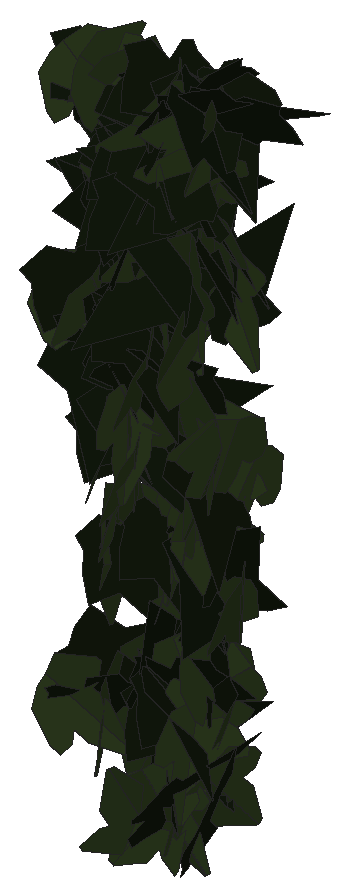
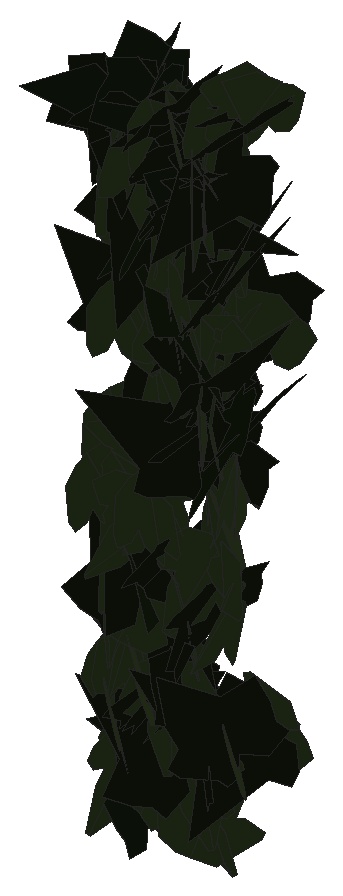
# SketchUp Ruby script. Lengths in inches.
U = 1.inch
M = Sketchup.active_model
def pt(a) = Geom::Point3d.new(a.map { |v| v * U })
def face(e, loops, mat)
  f = e.add_face(loops[0].map { |a| pt(a) })
  loops[1..].each { |l| e.add_face(l.map { |a| pt(a) }).erase! }
  f.material = f.back_material = mat if mat
  f
end
# faces: each face lists its corners as indices into pts; further lists are holes
def faces(e, pts, list, mat = nil) = list.each { |f| face(e, (f[0].is_a?(Array) ? f : [f]).map { |l| l.map { |i| pts[i] } }, mat) }
# xy, xz, yz: faces in a plane at the given z, y or x. An outline is a flat list of corners, or four numbers for a rectangle; further outlines are holes
def ring(l) = l.size == 4 ? [[l[0], l[1]], [l[2], l[1]], [l[2], l[3]], [l[0], l[3]]] : l.each_slice(2).to_a
def flat(e, list, mat, &to3) = list.each { |f| face(e, (f[0].is_a?(Array) ? f : [f]).map { |l| ring(l).map { |u, v| to3.(u, v) } }, mat) }
def xy(e, z, list, mat = nil) = flat(e, list, mat) { |x, y| [x, y, z] }
def xz(e, y, list, mat = nil) = flat(e, list, mat) { |x, z| [x, y, z] }
def yz(e, x, list, mat = nil) = flat(e, list, mat) { |y, z| [x, y, z] }
def lines(e, pts, list) = list.each { |a, b| e.add_line(pt(pts[a]), pt(pts[b])) }
# prism: a flat outline (further loops are holes) pulled along v
def prism(e, loops, v, mat = nil)
  f = face(e, loops, mat); d = Geom::Vector3d.new(v.map { |x| x * U })
  f.pushpull(f.normal.samedirection?(d) ? d.length : -d.length)
end
def box(e, o, s, mat = nil) = prism(e, [[o, [o[0] + s[0], o[1], o[2]], [o[0] + s[0], o[1] + s[1], o[2]], [o[0], o[1] + s[1], o[2]]]], [0, 0, s[2]], mat)
def at(x, y, z, deg = 0) = Geom::Transformation.translation(pt([x, y, z])) * Geom::Transformation.rotation(ORIGIN, Z_AXIS, deg.degrees)
def axes(o, x, y, z) = Geom::Transformation.new([*x, 0, *y, 0, *z, 0, *pt(o).to_a, 1])
def part(name) = M.definitions.add(name)
# library, detail: a bought-in or finely detailed component or shape, given as its bounding box
def library(name, o, s) = part(name).tap { |d| box(d.entities, o, s) }
def detail(e, o, s) = box(e.add_group.entities, o, s)
def put(e, d, t, mat = nil) = e.add_instance(d, t).tap { |i| i.material = mat if mat }
def group(e, t, mat = nil) = e.add_group.tap { |g| g.transformation = t; g.material = mat if mat }.entities
root = M.entities
M.materials.add("efeu1").color = [18, 25, 13]
M.materials.add("efeu2").color = [43, 57, 29]
c1 = part("ivyleaf_9")
p = [[1.54,2.16,1.25],[1.36,2.04,1.19],[-0.21,0.99,0.68],[-0.71,1.11,0.82],[-0.85,0.86,0.67],[-0.8,0.17,0.21],
  [-0.9,-0.01,0.1],[-0.67,-0.16,-0.02],[-0.08,-0.08,-0.05],[-0.03,-0.6,-0.4],[0.65,-0.88,-0.66],[0.83,-0.6,-0.49],
  [1.29,-0.42,-0.43],[1.8125,-0.07,-0.26],[1.21,0.44,0.15]]
faces(c1.entities,p,[[0,1,2,3,4,5,6,7,8,9,10,11,12,13,14]],"efeu1")
c2 = part("ivyleaf_10")
p = [[0,0.5,-0.03],[-0.0625,2.02,-0.43],[-0.19,2.01,-0.46],[-0.54,1.05,-0.29],[-0.52,0.625,-0.18],[-0.83,0.76,-0.28],
  [-1.16,0.64,-0.33],[-1.15,0.33,-0.24],[-0.77,-0.39,0.02],[-0.3,-0.51,0.16],[0.04,-0.48,0.23],[-0.02,2.01,-0.4375],
  [-0.06,2.01,-0.43],[0.04,-0.49,0.23],[0.67,-0.49,0.14],[1.38,0.36,-0.2],[1.375,0.51,-0.24],[0.81,0.65,-0.19],
  [0.62,0.59,-0.15],[0.6,1.09,-0.28],[0.5,1.23,-0.31]]
faces(c2.entities,p,[[0,1,2,3,4,5,6,7,8,9,10],[11,12,0,13,14,15,16,17,18,19,20]],"efeu2")
put(root,c1,axes([26.85,224.39,219.23],[0.01117,-0.47465,0.1568],[0.04061,-0.15546,-0.47348],[0.49822,0.02332,0.03508]))
put(root,c1,axes([27.04,224.61,221.03],[-0.15188,-0.0856,0.46862],[-0.11517,-0.47067,-0.1233],[0.46224,-0.14539,0.12325]))
put(root,c1,axes([26.95,224.09,215.43],[0.39928,0.30016,-0.02189],[-0.01757,-0.01306,-0.49952],[-0.30044,0.39967,0.00012]))
put(root,c1,axes([27.18,224.76,220.63],[-0.0054,-0.49964,0.01817],[0.00355,0.01813,0.49966],[-0.49996,0.00553,0.00335]))
put(root,c2,axes([27.07,224.33,216.95],[0.09969,-0.16852,-0.46007],[0.02423,0.47062,-0.16713],[0.48936,0.01103,0.102]))
put(root,c2,axes([26.68,223.98,215.4],[0.18664,0.05922,0.46006],[0.44103,0.13102,-0.19578],[-0.14374,0.47888,-0.00333]))
put(root,c2,axes([27.21,224.04,218.6],[0.07906,-0.26335,-0.41761],[-0.14047,0.39345,-0.27471],[0.47331,0.16076,-0.01177]))
put(root,c2,axes([26.77,223.9375,220.31],[0.2244,0.20804,0.39543],[0.29999,0.25778,-0.30587],[-0.33113,0.37452,-0.00912]))
put(root,c1,axes([27.27,224.71,219.45],[-0.16065,-0.47331,-0.01309],[0.01351,-0.0184,0.49948],[-0.47329,0.16013,0.0187]))
put(root,c1,axes([27.02,224.31,219.47],[0.40451,-0.11818,-0.26909],[-0.25817,0.07588,-0.42142],[0.14044,0.47987,0.00036]))
put(root,c1,axes([26.85,224.47,222.93],[0.08992,-0.48476,-0.0832],[0.07638,0.09732,-0.48445],[0.48588,0.07441,0.09155]))
put(root,c2,axes([26.92,223.96,223.06],[0.20217,0.37365,0.26366],[0.13517,0.22656,-0.42473],[-0.43687,0.24302,-0.0094]))
put(root,c2,axes([26.97,224.49,215.43],[0.2392,-0.318,0.30276],[0.20685,-0.22249,-0.39713],[0.38729,0.31524,0.02511]))
put(root,c1,axes([26.97,224.41,222.48],[0.41401,0.27531,0.05291],[0.05261,0.0164,-0.49695],[-0.27537,0.41705,-0.01538]))
put(root,c1,axes([27.01,224.29,221.35],[0.32908,-0.29569,-0.23296],[-0.17513,0.15365,-0.44241],[0.33322,0.37277,-0.00245]))
put(root,c2,axes([27.14,224,223.04],[0.03905,0.34792,0.35697],[-0.06235,0.35866,-0.34275],[-0.49456,-0.01775,0.0714]))
put(root,c1,axes([26.86,224.59,215.36],[-0.06324,-0.0071,0.49593],[0.49593,-0.00852,0.06312],[0.00755,0.49988,0.00812]))
put(root,c2,axes([27.15,223.96,220.41],[-0.05576,-0.45222,-0.20587],[0.08827,0.19486,-0.45193],[0.48898,-0.08675,0.0581]))
put(root,c2,axes([27.23,224.39,222.96],[-0.12269,-0.48418,-0.02274],[0.01304,0.02015,-0.49942],[0.48454,-0.12314,0.00768]))
put(root,c2,axes([27.11,224.31,217.375],[0.24025,-0.43764,0.02742],[-0.00015,0.03118,0.49903],[-0.4385,-0.23979,0.01485]))
put(root,c2,axes([27.18,224.18,219.97],[0.12548,0.34493,-0.33952],[0.05452,0.33844,0.36399],[0.48092,-0.12837,0.04733]))
put(root,c2,axes([27.1875,224.36,218.49],[-0.40365,0.29443,-0.01956],[0.01995,-0.00583,-0.49957],[-0.2944,-0.40408,-0.00704]))
put(root,c1,axes([26.99,223.91,220.76],[-0.03728,-0.1951,-0.45885],[0.14823,0.43499,-0.197],[0.47607,-0.15072,0.0254]))
put(root,c2,axes([27.37,224.56,219.68],[0.14882,-0.29129,-0.37816],[-0.15788,0.34378,-0.32694],[0.45048,0.21671,0.01034]))
put(root,c1,axes([27.07,224.55,217.21],[0.14098,-0.38613,-0.28466],[-0.06576,0.27834,-0.41013],[0.47519,0.15308,0.02769]))
put(root,c2,axes([27.2,224.64,217.57],[-0.47066,0.02713,-0.16655],[0.16675,-0.00077,-0.47137],[-0.02584,-0.49926,-0.00832]))
put(root,c1,axes([27.69,224.57,221.62],[-0.31695,0.07509,0.37935],[-0.3678,0.09296,-0.3257],[-0.11944,-0.48551,-0.00369]))
put(root,c2,axes([27.46,224.375,222.32],[0.10723,-0.23008,-0.43077],[-0.18386,0.38957,-0.25384],[0.45244,0.21284,-0.00106]))
put(root,c2,axes([27.34,224.65,222.26],[0.18297,-0.41234,-0.21564],[-0.02654,0.22209,-0.44718],[0.46456,0.17509,0.05938]))
put(root,c2,axes([27.53,224.14,221.58],[-0.43573,-0.03493,0.24274],[-0.23476,-0.08372,-0.43345],[0.07092,-0.4917,0.05656]))
put(root,c2,axes([27.43,224.72,220.42],[-0.37069,-0.33552,-0.00391],[0.00268,0.00286,-0.49998],[0.33553,-0.3707,-0.00032]))
put(root,c2,axes([27.13,224.6,219.23],[0.12946,-0.18409,0.44649],[0.35029,-0.28243,-0.21802],[0.33247,0.36925,0.05584]))
put(root,c2,axes([27.6,224.45,214.96],[-0.43721,-0.08452,0.22738],[-0.22603,-0.0282,-0.4451],[0.08806,-0.492,-0.01354]))
put(root,c1,axes([27.47,224.68,221.95],[-0.30706,-0.36456,0.15104],[-0.06968,-0.13828,-0.47542],[0.38841,-0.31301,0.03411]))
put(root,c1,axes([27.24,224.49,220.04],[0.24011,0.38946,0.20166],[-0.09867,-0.17604,0.45746],[0.42733,-0.25948,-0.00768]))
put(root,c1,axes([27.38,224.7,221.93],[-0.1233,-0.48443,-0.01097],[0.00351,0.01043,-0.49988],[0.48455,-0.12335,0.00083]))
put(root,c1,axes([27.14,224.02,219.74],[0.14993,-0.00016,0.47699],[0.46626,0.10549,-0.14652],[-0.10059,0.48874,0.03178]))
put(root,c2,axes([27.6,224.29,213.94],[-0.31895,-0.30639,-0.23322],[-0.14845,-0.18158,0.44158],[-0.35529,0.35093,0.02487]))
put(root,c1,axes([27.26,224.33,218.83],[-0.07244,-0.21034,-0.44778],[0.24746,0.37647,-0.21687],[0.42839,-0.25304,0.04955]))
put(root,c1,axes([27.74,224.66,220.78],[-0.30694,0.38374,-0.09236],[0.0627,-0.06812,-0.49135],[-0.38969,-0.31322,-0.0063]))
put(root,c2,axes([27.57,224.55,222.18],[0.43746,-0.22631,-0.08611],[-0.07205,0.04811,-0.49244],[0.23117,0.44325,0.00948]))
put(root,c1,axes([27.34,224.35,218.97],[0.08608,-0.41446,-0.2661],[0.03378,0.27447,-0.41656],[0.49137,0.05374,0.07525]))
put(root,c1,axes([27.76,223.86,221.32],[-0.16232,0.11742,-0.45811],[-0.3551,0.28962,0.20006],[0.31234,0.3903,-0.01063]))
put(root,c1,axes([27.47,224.74,222.625],[-0.1058,-0.48794,-0.02681],[0.00877,0.02553,-0.49927],[0.4886,-0.10612,0.00316]))
put(root,c2,axes([27.61,224,218.45],[0.11883,-0.46018,-0.15528],[0.00502,0.16101,-0.47334],[0.48565,0.11093,0.04288]))
put(root,c1,axes([27.75,224.34,222.58],[-0.42684,0.21247,-0.15055],[0.13313,-0.07039,-0.47678],[-0.2238,-0.4471,0.00352]))
put(root,c2,axes([27.73,224.61,215.88],[-0.48549,-0.0978,0.06878],[-0.06745,-0.01346,-0.49525],[0.09872,-0.49016,-0.00012]))
put(root,c2,axes([27.58,224.05,219.09],[0.07016,0.47942,-0.12341],[-0.03957,-0.11881,-0.48406],[-0.49347,0.07769,0.02127]))
put(root,c2,axes([27.68,224.54,217.03],[0.28528,-0.39847,-0.09918],[-0.05978,0.07917,-0.49006],[0.40625,0.29147,-0.00247]))
put(root,c2,axes([27.68,224.68,220.875],[0.36148,-0.31601,-0.13952],[-0.05411,0.14766,-0.47463],[0.34118,0.35823,0.07255]))
put(root,c2,axes([27.61,224.89,220.81],[0.0394,-0.16562,0.47013],[0.10887,-0.45735,-0.17024],[0.48641,0.11578,0.00002]))
put(root,c2,axes([27.73,224.05,219.65],[0.09976,-0.42101,-0.2506],[-0.04747,0.24623,-0.43257],[0.48764,0.11009,0.00916]))
put(root,c1,axes([27.36,224.56,215.13],[-0.03342,-0.01638,-0.49861],[0.49822,-0.02689,-0.03251],[-0.02575,-0.49901,0.01812]))
put(root,c1,axes([27.59,224.55,215.7],[0.08273,0.26611,0.41514],[-0.16662,-0.38109,0.27749],[0.4641,-0.18426,0.02563]))
put(root,c2,axes([27.41,224.6875,220.49],[0.24588,-0.20678,0.38313],[0.34647,-0.1735,-0.316],[0.26363,0.42088,0.05797]))
put(root,c2,axes([27.84,224.19,214.32],[0.41234,-0.12911,-0.25162],[-0.24284,0.06635,-0.432],[0.14494,0.47847,-0.00799]))
put(root,c1,axes([27.51,224.27,220.16],[0.10713,-0.4709,-0.12954],[-0.00593,0.13136,-0.4824],[0.48835,0.10489,0.02256]))
put(root,c2,axes([27.73,224.51,222.79],[0.23082,-0.44348,-0.00653],[-0.00185,0.0064,-0.49996],[0.44353,0.23083,0.00132]))
put(root,c2,axes([27.86,224.24,222.31],[-0.37407,-0.3261,0.06105],[-0.04322,-0.04332,-0.49624],[0.32894,-0.37654,0.00423]))
put(root,c1,axes([27.89,224.13,219.61],[0.2048,0.31369,-0.33114],[-0.18044,-0.27767,-0.37462],[-0.41893,0.27295,-0.00053]))
put(root,c1,axes([27.375,224.67,218.78],[0.10284,-0.03814,0.48782],[0.47965,-0.09071,-0.10821],[0.09676,0.49022,0.01793]))
put(root,c1,axes([27.64,224.33,222.17],[-0.08263,-0.42112,-0.25658],[0.03457,0.25457,-0.42895],[0.49191,-0.08863,-0.01295]))
put(root,c2,axes([27.84,224.83,218.28],[-0.17138,-0.4468,0.14489],[0.00794,-0.15697,-0.47466],[0.46964,-0.16039,0.0609]))
put(root,c2,axes([28.03,224.4,220.84],[0.16934,-0.18519,-0.43247],[-0.22363,0.3727,-0.24716],[0.4139,0.27713,0.0434]))
put(root,c1,axes([27.67,224.53,217.57],[0.09946,-0.44972,-0.19458],[-0.03311,0.19193,-0.46051],[0.48889,0.10449,0.00839]))
put(root,c1,axes([27.65,224.61,222.99],[0.10473,-0.47967,-0.0946],[-0.00259,0.0962,-0.49065],[0.4889,0.10326,0.01767]))
put(root,c1,axes([27.72,224.68,222.73],[-0.14991,-0.47105,-0.07511],[0.10029,0.04585,-0.48769],[0.46634,-0.16128,0.08074]))
put(root,c1,axes([28.09,224.23,220.9],[-0.47101,-0.13344,0.10171],[-0.09635,-0.03302,-0.48952],[0.13736,-0.48073,0.00539]))
put(root,c2,axes([27.84,224.53,218.5],[-0.36173,-0.34361,0.03299],[0.02646,0.02004,0.4989],[-0.34417,0.36267,0.00369]))
put(root,c2,axes([27.92,224.1875,221.05],[-0.24814,-0.43206,-0.04187],[0.01715,0.03843,-0.49823],[0.43374,-0.2487,-0.00425]))
put(root,c2,axes([27.93,224.59,222.71],[-0.06891,-0.48036,0.12045],[0.01082,-0.12304,-0.4845],[0.49511,-0.06417,0.02735]))
put(root,c2,axes([27.96,224.29,219.4375],[-0.47465,0.15718,-0.00058],[0.0002,-0.00122,-0.5],[-0.15718,-0.47465,0.0011]))
put(root,c1,axes([27.5625,224.68,215.02],[0.38011,0.24524,-0.213],[0.17405,0.12305,0.45229],[0.27426,-0.41799,0.00818]))
put(root,c1,axes([27.95,224.52,221.69],[0.27643,0.41421,-0.04487],[-0.02059,-0.0402,-0.49796],[-0.41613,0.27715,-0.00517]))
put(root,c2,axes([28.01,224.68,222.3],[-0.28969,-0.40566,0.03897],[0.02606,-0.06615,-0.49492],[0.4067,-0.28471,0.05947]))
put(root,c1,axes([27.82,224.08,221.75],[-0.10442,-0.39438,-0.28907],[0.06537,0.28168,-0.4079],[0.48459,-0.12298,-0.00727]))
put(root,c1,axes([28.15,224.36,222.94],[0.02001,0.4946,-0.07051],[-0.02127,-0.06966,-0.49467],[-0.49915,0.0228,0.01825]))
put(root,c1,axes([27.85,224.4,215.75],[0.18587,-0.4069,-0.22336],[-0.0869,0.20584,-0.4473],[0.45596,0.2051,0.0058]))
put(root,c2,axes([28.17,224.77,216.59],[-0.44103,-0.14302,-0.18718],[-0.17109,-0.07861,0.46319],[-0.16192,0.47262,0.0204]))
put(root,c2,axes([27.96,224.42,217.8],[0.41058,-0.27437,0.07839],[0.06825,-0.03894,-0.49379],[0.27707,0.41618,0.00547]))
put(root,c1,axes([28.125,224.63,221.86],[-0.31371,-0.30816,0.23797],[-0.1029,-0.22911,-0.43234],[0.3755,-0.32023,0.08033]))
put(root,c1,axes([27.89,224.42,215.64],[0.01016,-0.36796,-0.33838],[-0.00999,0.33823,-0.3681],[0.4998,0.01424,-0.00048]))
put(root,c1,axes([28.33,224.41,215.74],[0.01955,-0.04863,0.49725],[-0.29553,0.40011,0.05075],[-0.40284,-0.29589,-0.0131]))
put(root,c1,axes([28.45,224.16,222.09],[-0.29052,0.1168,0.38982],[-0.39346,0.04161,-0.30571],[-0.10386,-0.48438,0.06773]))
put(root,c2,axes([28.13,224.93,220.57],[-0.20779,-0.40735,0.20221],[-0.02015,-0.21385,-0.45151],[0.45433,-0.19579,0.07246]))
put(root,c2,axes([27.79,224.61,220.47],[0.38144,-0.07993,0.31323],[0.30755,-0.05952,-0.38971],[0.09959,0.48997,0.00376]))
put(root,c2,axes([28.22,224.55,216.13],[-0.35907,-0.31419,0.14951],[-0.10017,-0.1124,-0.47679],[0.33322,-0.37236,0.01777]))
put(root,c2,axes([27.88,224.12,214.59],[-0.39389,0.05915,-0.30224],[0.286,-0.11177,-0.3946],[-0.11425,-0.48374,0.05422]))
put(root,c1,axes([28.03,224.2,216.02],[0.41721,0.24579,-0.1246],[-0.10665,-0.06443,-0.48422],[-0.25409,0.43062,-0.00133]))
put(root,c1,axes([28.35,224.27,216.91],[-0.06569,0.27643,0.41142],[-0.10781,0.39712,-0.28403],[-0.4838,-0.12602,0.00743]))
put(root,c1,axes([27.8125,224.45,215.61],[0.20332,-0.40448,0.21226],[0.11442,-0.17983,-0.45229],[0.44223,0.23249,0.01944]))
put(root,c2,axes([27.98,224.83,218.11],[-0.43597,-0.06913,-0.23484],[0.24471,-0.13635,-0.41416],[-0.00678,-0.47606,0.15272]))
put(root,c2,axes([28.1,224.5625,214.38],[-0.10005,-0.24908,-0.42184],[-0.02826,-0.42689,0.25877],[-0.48907,0.07562,0.07134]))
put(root,c2,axes([28.17,224.63,221.29],[-0.45012,0.21703,0.01705],[-0.01597,0.00613,-0.49971],[-0.21711,-0.4504,0.00142]))
put(root,c2,axes([27.99,224.73,215.64],[0.34932,-0.32669,-0.14578],[0.10473,-0.10144,0.47827],[-0.34207,-0.36467,-0.00245]))
put(root,c2,axes([28.24,224.42,222.5],[-0.13071,-0.41524,0.24594],[-0.02135,-0.24958,-0.43273],[0.48214,-0.12362,0.04752]))
put(root,c2,axes([28.31,224.31,218.43],[0.30976,-0.26266,-0.29165],[-0.18355,0.23146,-0.4034],[0.34693,0.35698,0.04697]))
put(root,c2,axes([27.94,224.66,218.73],[0.35657,0.22716,0.26694],[0.20931,0.16744,-0.42208],[-0.28115,0.41275,0.02431]))
put(root,c1,axes([27.96,224.72,221.58],[0.38749,-0.3098,-0.06224],[-0.05556,0.03016,-0.49599],[0.31107,0.3913,-0.01105]))
put(root,c2,axes([28.47,224.61,215.93],[-0.21197,-0.17599,0.41725],[-0.25888,-0.3309,-0.27108],[0.37155,-0.33096,0.04916]))
put(root,c2,axes([28.15,224.22,220.67],[-0.46082,0.06537,0.18269],[0.17617,-0.05638,0.46453],[0.08133,0.49249,0.02893]))
put(root,c2,axes([28.19,224.31,217.57],[0.02071,0.12393,0.48396],[-0.02662,0.48396,-0.12279],[-0.49886,-0.02068,0.02664]))
put(root,c2,axes([28.37,224.28,222.11],[-0.33911,-0.34432,0.12826],[-0.08009,-0.10107,-0.48308],[0.3586,-0.34818,0.01339]))
put(root,c2,axes([28.36,223.74,219.93],[0.08535,-0.14214,0.47171],[-0.22495,0.41467,0.16566],[-0.4383,-0.24051,0.00684]))
put(root,c1,axes([28.13,223.68,214.53],[-0.03234,0.4584,-0.19703],[-0.01465,0.19648,0.45954],[0.49874,0.03549,0.00073]))
put(root,c2,axes([28.33,224.83,215.57],[0.2486,-0.433,-0.0267],[-0.01276,0.02347,-0.49929],[0.43363,0.24892,0.00062]))
put(root,c2,axes([28.37,224.65,221.73],[-0.01245,-0.49711,-0.05217],[-0.00953,0.05242,-0.49715],[0.49975,-0.01139,-0.01078]))
put(root,c1,axes([28.14,224.66,222.83],[-0.06785,-0.39256,-0.30215],[0.09694,0.28855,-0.39666],[0.4858,-0.11241,0.03695]))
put(root,c2,axes([28.29,224.25,215.4],[0.13381,0.45743,-0.15116],[-0.05001,-0.14285,-0.47654],[-0.47916,0.14265,0.00752]))
put(root,c1,axes([28.0625,224.75,216.95],[0.49392,0.04723,-0.06173],[0.0525,0.09011,0.489],[0.05732,-0.48954,0.08406]))
put(root,c2,axes([28.38,224.15,216.27],[-0.06766,0.32854,0.37078],[-0.11456,0.35371,-0.33432],[-0.48197,-0.13019,0.02741]))
put(root,c1,axes([28.23,224.41,213.97],[0.04762,0.39664,0.30068],[-0.06435,-0.29461,0.39883],[0.49355,-0.07668,0.02299]))
put(root,c1,axes([28.19,224.49,216.99],[0.02153,-0.31971,0.38383],[0.03553,-0.38223,-0.32037],[0.49827,0.04107,0.00626]))
put(root,c1,axes([28.24,224.52,220.29],[-0.163,-0.07758,0.46627],[0.44743,0.13375,0.17867],[-0.15245,0.47549,0.02582]))
put(root,c1,axes([28.27,224.13,223],[0.35329,-0.28672,-0.20732],[-0.16086,0.13079,-0.45499],[0.31514,0.38818,0.00018]))
put(root,c1,axes([28.11,224.54,221.07],[0.14693,-0.33398,0.34186],[0.18565,-0.28968,-0.36279],[0.44039,0.23354,0.03889]))
put(root,c2,axes([28.47,224.92,218.34],[-0.14696,-0.40958,0.24626],[0.04102,-0.26751,-0.42043],[0.47615,-0.10337,0.11223]))
put(root,c1,axes([28.55,224.44,222.88],[0.27507,0.32218,-0.26558],[-0.21732,-0.16109,-0.4205],[-0.35652,0.34677,0.05141]))
put(root,c2,axes([28.42,224.38,214.73],[-0.14572,-0.36092,-0.31385],[0.11969,0.29014,-0.38922],[0.46308,-0.18857,0.00184]))
put(root,c2,axes([28.38,224.53,222.59],[-0.03382,0.19405,-0.45957],[0.02375,-0.45947,-0.19576],[-0.49829,-0.03507,0.02186]))
put(root,c2,axes([28.54,224.51,218.88],[-0.15028,-0.46381,0.11086],[-0.01246,-0.11238,-0.48705],[0.47672,-0.14915,0.02222]))
put(root,c2,axes([28.46,224.39,218.78],[0.07662,-0.41444,0.26901],[0.09627,-0.25449,-0.41949],[0.48462,0.11608,0.0408]))
put(root,c2,axes([28.55,224.6,216.96],[0.12934,-0.45132,-0.17198],[-0.00931,0.17568,-0.46803],[0.48289,0.12427,0.03704]))
put(root,c2,axes([28.22,224.76,220.55],[0.37561,-0.00031,0.33002],[0.33,0.0059,-0.37558],[-0.00366,0.49997,0.00463]))
put(root,c1,axes([28.29,224.46,218.36],[0.09844,-0.45386,0.18525],[0.05782,-0.17688,-0.46408],[0.48679,0.11279,0.01766]))
put(root,c1,axes([28.17,224.3,222.75],[0.34594,-0.08303,0.35132],[0.35716,0.14955,-0.31635],[-0.05255,0.46983,0.16278]))
